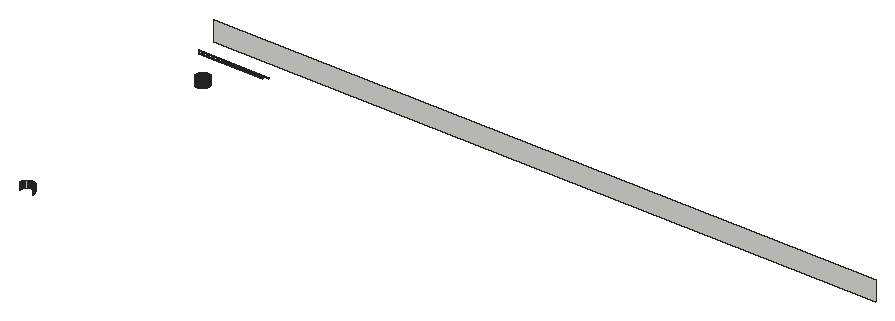
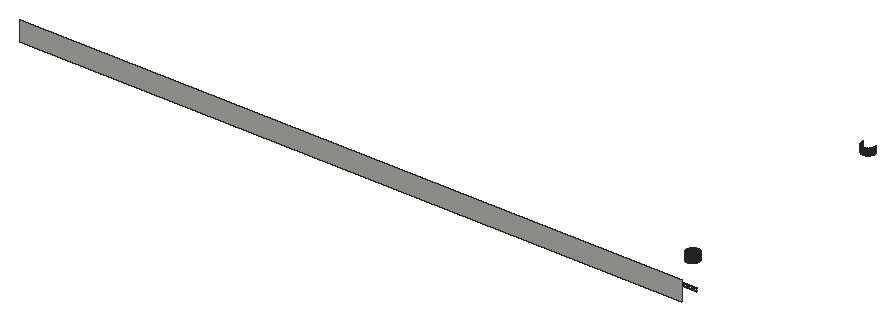
# SketchUp Ruby script. Lengths in inches.
U = 1.inch
M = Sketchup.active_model
def pt(a) = Geom::Point3d.new(a.map { |v| v * U })
def face(e, loops, mat)
  f = e.add_face(loops[0].map { |a| pt(a) })
  loops[1..].each { |l| e.add_face(l.map { |a| pt(a) }).erase! }
  f.material = f.back_material = mat if mat
  f
end
# faces: each face lists its corners as indices into pts; further lists are holes
def faces(e, pts, list, mat = nil) = list.each { |f| face(e, (f[0].is_a?(Array) ? f : [f]).map { |l| l.map { |i| pts[i] } }, mat) }
# xy, xz, yz: faces in a plane at the given z, y or x. An outline is a flat list of corners, or four numbers for a rectangle; further outlines are holes
def ring(l) = l.size == 4 ? [[l[0], l[1]], [l[2], l[1]], [l[2], l[3]], [l[0], l[3]]] : l.each_slice(2).to_a
def flat(e, list, mat, &to3) = list.each { |f| face(e, (f[0].is_a?(Array) ? f : [f]).map { |l| ring(l).map { |u, v| to3.(u, v) } }, mat) }
def xy(e, z, list, mat = nil) = flat(e, list, mat) { |x, y| [x, y, z] }
def xz(e, y, list, mat = nil) = flat(e, list, mat) { |x, z| [x, y, z] }
def yz(e, x, list, mat = nil) = flat(e, list, mat) { |y, z| [x, y, z] }
def lines(e, pts, list) = list.each { |a, b| e.add_line(pt(pts[a]), pt(pts[b])) }
# prism: a flat outline (further loops are holes) pulled along v
def prism(e, loops, v, mat = nil)
  f = face(e, loops, mat); d = Geom::Vector3d.new(v.map { |x| x * U })
  f.pushpull(f.normal.samedirection?(d) ? d.length : -d.length)
end
def box(e, o, s, mat = nil) = prism(e, [[o, [o[0] + s[0], o[1], o[2]], [o[0] + s[0], o[1] + s[1], o[2]], [o[0], o[1] + s[1], o[2]]]], [0, 0, s[2]], mat)
def at(x, y, z, deg = 0) = Geom::Transformation.translation(pt([x, y, z])) * Geom::Transformation.rotation(ORIGIN, Z_AXIS, deg.degrees)
def axes(o, x, y, z) = Geom::Transformation.new([*x, 0, *y, 0, *z, 0, *pt(o).to_a, 1])
def part(name) = M.definitions.add(name)
# library, detail: a bought-in or finely detailed component or shape, given as its bounding box
def library(name, o, s) = part(name).tap { |d| box(d.entities, o, s) }
def detail(e, o, s) = box(e.add_group.entities, o, s)
def put(e, d, t, mat = nil) = e.add_instance(d, t).tap { |i| i.material = mat if mat }
def group(e, t, mat = nil) = e.add_group.tap { |g| g.transformation = t; g.material = mat if mat }.entities
root = M.entities
xz(root,437.5,[[30.34,129,30.42,132],[30.42,129,30.5,132],[30.5,129,30.58,132],[30.58,129,30.66,132]])
xz(root,534,[[30.34,129,30.42,132],[30.42,129,30.5,132],[30.5,129,30.58,132],[30.58,129,30.66,132]])
xz(root,540,[[30.34,129,30.42,132],[30.42,129,30.5,132],[30.5,129,30.58,132],[30.58,129,30.66,132]])
xz(root,553.5,[[15.5,129,45.5,129.5]])
xz(root,555,[[14,129,47,129.5]])
xz(root,564,[[14,129,323,138]])
yz(root,27.5,[[434.34,129,434.42,132],[434.42,129,434.5,132],[434.5,129,434.58,132],[434.58,129,434.66,132],[536.84,129,536.92,132],
  [536.92,129,537,132],[537,129,537.08,132],[537.08,129,537.16,132]])
yz(root,33.5,[[434.34,129,434.42,132],[434.42,129,434.5,132],[434.5,129,434.58,132],[434.58,129,434.66,132],[536.84,129,536.92,132],
  [536.92,129,537,132],[537,129,537.08,132],[537.08,129,537.16,132]])
p = [[27.57,433.875,129],[27.55,433.95,129],[27.55,433.95,132],[27.57,433.875,132],[33.45,433.95,129],[33.43,433.875,129],
  [33.43,433.875,132],[33.45,433.95,132],[27.54,434.03,129],[27.54,434.03,132],[27.53,434.11,129],[27.53,434.11,132],
  [33.46,434.03,129],[33.46,434.03,132],[33.47,434.11,129],[33.47,434.11,132],[27.52,434.1875,129],[27.52,434.1875,132],
  [33.48,434.1875,129],[33.48,434.1875,132],[27.51,434.26,129],[27.51,434.26,132],[33.49,434.26,129],[33.49,434.26,132],
  [27.5,434.34,129],[27.5,434.34,132],[33.5,434.34,129],[33.5,434.34,132],[27.5,434.66,129],[27.51,434.74,129],
  [27.51,434.74,132],[27.5,434.66,132],[27.52,434.8125,129],[27.52,434.8125,132],[33.49,434.74,129],[33.5,434.66,129],
  [33.5,434.66,132],[33.49,434.74,132],[33.48,434.8125,129],[33.48,434.8125,132],[27.53,434.89,129],[27.53,434.89,132],
  [33.47,434.89,129],[33.47,434.89,132],[27.54,434.97,129],[27.54,434.97,132],[33.46,434.97,129],[33.46,434.97,132],
  [27.55,435.05,129],[27.55,435.05,132],[27.57,435.125,129],[27.57,435.125,132],[33.45,435.05,129],[33.45,435.05,132],
  [33.43,435.125,129],[33.43,435.125,132],[27.58,435.2,129],[27.58,435.2,132],[33.42,435.2,129],[33.42,435.2,132],
  [27.6,435.28,129],[27.6,435.28,132],[33.4,435.28,129],[33.4,435.28,132],[27.625,435.35,129],[27.625,435.35,132],
  [33.375,435.35,129],[33.375,435.35,132],[27.65,435.43,129],[27.65,435.43,132],[27.67,435.5,129],[27.67,435.5,132],
  [33.33,435.5,129],[33.35,435.43,129],[33.35,435.43,132],[33.33,435.5,132],[27.7,435.58,129],[27.7,435.58,132],
  [33.3,435.58,129],[33.3,435.58,132],[27.73,435.65,129],[27.73,435.65,132],[27.76,435.72,129],[27.76,435.72,132],
  [33.24,435.72,129],[33.27,435.65,129],[33.27,435.65,132],[33.24,435.72,132],[27.79,435.79,129],[27.79,435.79,132],
  [33.21,435.79,129],[33.21,435.79,132],[27.83,435.86,129],[27.83,435.86,132],[33.17,435.86,129],[33.17,435.86,132],
  [27.86,435.93,129],[27.86,435.93,132],[27.9,436,129],[27.9,436,132],[33.14,435.93,129],[33.14,435.93,132],
  [33.1,436,129],[33.1,436,132],[27.94,436.07,129],[27.94,436.07,132],[33.06,436.07,129],[33.06,436.07,132],
  [27.98,436.13,129],[27.98,436.13,132],[28.03,436.2,129],[28.03,436.2,132],[33.02,436.13,129],[33.02,436.13,132],
  [32.97,436.2,129],[32.97,436.2,132],[28.07,436.26,129],[28.07,436.26,132],[32.93,436.26,129],[32.93,436.26,132],
  [28.12,436.33,129],[28.12,436.33,132],[28.17,436.39,129],[28.17,436.39,132],[32.83,436.39,129],[32.88,436.33,129],
  [32.88,436.33,132],[32.83,436.39,132],[28.22,436.45,129],[28.22,436.45,132],[28.27,436.51,129],[28.27,436.51,132],
  [32.73,436.51,129],[32.78,436.45,129],[32.78,436.45,132],[32.73,436.51,132],[28.32,436.57,129],[28.32,436.57,132],
  [32.68,436.57,129],[32.68,436.57,132],[28.38,436.62,129],[28.38,436.62,132],[28.43,436.68,129],[28.43,436.68,132],
  [32.62,436.62,129],[32.62,436.62,132],[32.57,436.68,129],[32.57,436.68,132],[28.49,436.73,129],[28.49,436.73,132],
  [28.55,436.78,129],[28.55,436.78,132],[32.45,436.78,129],[32.51,436.73,129],[32.51,436.73,132],[32.45,436.78,132],
  [28.61,436.83,129],[28.61,436.83,132],[28.67,436.88,129],[28.67,436.88,132],[32.33,436.88,129],[32.39,436.83,129],
  [32.39,436.83,132],[32.33,436.88,132],[28.74,436.93,129],[28.74,436.93,132],[28.8,436.97,129],[28.8,436.97,132],
  [32.2,436.97,129],[32.26,436.93,129],[32.26,436.93,132],[32.2,436.97,132],[28.87,437.02,129],[28.87,437.02,132],
  [28.93,437.06,129],[28.93,437.06,132],[32.13,437.02,129],[32.13,437.02,132],[32.07,437.06,129],[32.07,437.06,132],
  [29,437.1,129],[29,437.1,132],[29.07,437.14,129],[29.07,437.14,132],[29.14,437.17,129],[29.14,437.17,132],
  [31.93,437.14,129],[32,437.1,129],[32,437.1,132],[31.93,437.14,132],[31.86,437.17,129],[31.86,437.17,132],
  [29.21,437.21,129],[29.21,437.21,132],[29.28,437.24,129],[29.28,437.24,132],[29.35,437.27,129],[29.35,437.27,132],
  [31.65,437.27,129],[31.72,437.24,129],[31.72,437.24,132],[31.65,437.27,132],[31.79,437.21,129],[31.79,437.21,132],
  [29.42,437.3,129],[29.42,437.3,132],[29.5,437.33,129],[29.5,437.33,132],[29.57,437.35,129],[29.57,437.35,132],
  [31.43,437.35,129],[31.5,437.33,129],[31.5,437.33,132],[31.43,437.35,132],[31.58,437.3,129],[31.58,437.3,132],
  [29.65,437.375,129],[29.65,437.375,132],[29.72,437.4,129],[29.72,437.4,132],[29.8,437.42,129],[29.8,437.42,132],
  [29.875,437.43,129],[29.875,437.43,132],[29.95,437.45,129],[29.95,437.45,132],[30.03,437.46,129],[30.03,437.46,132],
  [31.05,437.45,129],[31.125,437.43,129],[31.125,437.43,132],[31.05,437.45,132],[30.97,437.46,129],[30.97,437.46,132],
  [31.2,437.42,129],[31.2,437.42,132],[31.28,437.4,129],[31.28,437.4,132],[31.35,437.375,129],[31.35,437.375,132],
  [30.11,437.47,129],[30.11,437.47,132],[30.1875,437.48,129],[30.1875,437.48,132],[30.26,437.49,129],[30.26,437.49,132],
  [30.34,437.5,129],[30.34,437.5,132],[30.74,437.49,129],[30.8125,437.48,129],[30.8125,437.48,132],[30.74,437.49,132],
  [30.66,437.5,129],[30.66,437.5,132],[30.89,437.47,129],[30.89,437.47,132],[30.11,534.03,129],[30.03,534.04,129],
  [30.03,534.04,132],[30.11,534.03,132],[29.95,534.05,129],[29.95,534.05,132],[30.1875,534.02,129],[30.1875,534.02,132],
  [30.26,534.01,129],[30.26,534.01,132],[30.34,534,129],[30.34,534,132],[30.74,534.01,129],[30.66,534,129],
  [30.66,534,132],[30.74,534.01,132],[30.8125,534.02,129],[30.8125,534.02,132],[30.89,534.03,129],[30.89,534.03,132],
  [30.97,534.04,129],[30.97,534.04,132],[31.05,534.05,129],[31.05,534.05,132],[29.57,534.15,129],[29.5,534.17,129],
  [29.5,534.17,132],[29.57,534.15,132],[29.72,534.1,129],[29.65,534.125,129],[29.65,534.125,132],[29.72,534.1,132],
  [29.8,534.08,129],[29.8,534.08,132],[29.875,534.07,129],[29.875,534.07,132],[31.125,534.07,129],[31.125,534.07,132],
  [31.2,534.08,129],[31.2,534.08,132],[31.28,534.1,129],[31.28,534.1,132],[31.35,534.125,129],[31.35,534.125,132],
  [31.43,534.15,129],[31.43,534.15,132],[31.5,534.17,129],[31.5,534.17,132],[29.35,534.23,129],[29.28,534.26,129],
  [29.28,534.26,132],[29.35,534.23,132],[29.42,534.2,129],[29.42,534.2,132],[31.58,534.2,129],[31.58,534.2,132],
  [31.65,534.23,129],[31.65,534.23,132],[31.72,534.26,129],[31.72,534.26,132],[29.21,534.29,129],[29.14,534.33,129],
  [29.14,534.33,132],[29.21,534.29,132],[29.07,534.36,129],[29.07,534.36,132],[31.79,534.29,129],[31.79,534.29,132],
  [31.86,534.33,129],[31.86,534.33,132],[31.93,534.36,129],[31.93,534.36,132],[29,534.4,129],[28.93,534.44,129],
  [28.93,534.44,132],[29,534.4,132],[28.87,534.48,129],[28.87,534.48,132],[32,534.4,129],[32,534.4,132],
  [32.07,534.44,129],[32.07,534.44,132],[32.13,534.48,129],[32.13,534.48,132],[28.8,534.53,129],[28.74,534.57,129],
  [28.74,534.57,132],[28.8,534.53,132],[32.2,534.53,129],[32.2,534.53,132],[32.26,534.57,129],[32.26,534.57,132],
  [28.67,534.62,129],[28.61,534.67,129],[28.61,534.67,132],[28.67,534.62,132],[32.33,534.62,129],[32.33,534.62,132],
  [32.39,534.67,129],[32.39,534.67,132],[28.55,534.72,129],[28.49,534.77,129],[28.49,534.77,132],[28.55,534.72,132],
  [32.45,534.72,129],[32.45,534.72,132],[32.51,534.77,129],[32.51,534.77,132],[28.43,534.82,129],[28.43,534.82,132],
  [28.38,534.88,129],[28.38,534.88,132],[32.57,534.82,129],[32.57,534.82,132],[32.62,534.88,129],[32.62,534.88,132],
  [28.32,534.93,129],[28.32,534.93,132],[28.27,534.99,129],[28.27,534.99,132],[32.68,534.93,129],[32.68,534.93,132],
  [32.73,534.99,129],[32.73,534.99,132],[28.22,535.05,129],[28.22,535.05,132],[32.78,535.05,129],[32.78,535.05,132],
  [28.17,535.11,129],[28.12,535.17,129],[28.12,535.17,132],[28.17,535.11,132],[32.83,535.11,129],[32.83,535.11,132],
  [32.88,535.17,129],[32.88,535.17,132],[28.07,535.24,129],[28.03,535.3,129],[28.03,535.3,132],[28.07,535.24,132],
  [32.93,535.24,129],[32.93,535.24,132],[32.97,535.3,129],[32.97,535.3,132],[27.98,535.37,129],[27.98,535.37,132],
  [33.02,535.37,129],[33.02,535.37,132],[27.94,535.43,129],[27.94,535.43,132],[27.9,535.5,129],[27.9,535.5,132],
  [33.06,535.43,129],[33.06,535.43,132],[33.1,535.5,129],[33.1,535.5,132],[27.86,535.57,129],[27.86,535.57,132],
  [33.14,535.57,129],[33.14,535.57,132],[27.83,535.64,129],[27.83,535.64,132],[27.79,535.71,129],[27.79,535.71,132],
  [33.17,535.64,129],[33.17,535.64,132],[33.21,535.71,129],[33.21,535.71,132],[27.76,535.78,129],[27.76,535.78,132],
  [33.24,535.78,129],[33.24,535.78,132],[27.73,535.85,129],[27.73,535.85,132],[33.27,535.85,129],[33.27,535.85,132],
  [27.7,535.92,129],[27.7,535.92,132],[27.67,536,129],[27.67,536,132],[33.3,535.92,129],[33.3,535.92,132],
  [33.33,536,129],[33.33,536,132],[27.65,536.07,129],[27.65,536.07,132],[33.35,536.07,129],[33.35,536.07,132],
  [27.625,536.15,129],[27.625,536.15,132],[27.6,536.22,129],[27.6,536.22,132],[33.375,536.15,129],[33.375,536.15,132],
  [33.4,536.22,129],[33.4,536.22,132],[27.58,536.3,129],[27.58,536.3,132],[33.42,536.3,129],[33.42,536.3,132],
  [27.57,536.375,129],[27.57,536.375,132],[33.43,536.375,129],[33.43,536.375,132],[27.55,536.45,129],[27.55,536.45,132],
  [33.45,536.45,129],[33.45,536.45,132],[27.54,536.53,129],[27.54,536.53,132],[27.53,536.61,129],[27.53,536.61,132],
  [33.46,536.53,129],[33.46,536.53,132],[33.47,536.61,129],[33.47,536.61,132],[27.52,536.6875,129],[27.52,536.6875,132],
  [33.48,536.6875,129],[33.48,536.6875,132],[27.51,536.76,129],[27.51,536.76,132],[33.49,536.76,129],[33.49,536.76,132],
  [27.5,536.84,129],[27.5,536.84,132],[33.5,536.84,129],[33.5,536.84,132],[27.5,537.16,129],[27.51,537.24,129],
  [27.51,537.24,132],[27.5,537.16,132],[27.52,537.3125,129],[27.52,537.3125,132],[33.49,537.24,129],[33.5,537.16,129],
  [33.5,537.16,132],[33.49,537.24,132],[33.48,537.3125,129],[33.48,537.3125,132],[27.53,537.39,129],[27.53,537.39,132],
  [33.47,537.39,129],[33.47,537.39,132],[27.54,537.47,129],[27.54,537.47,132],[33.46,537.47,129],[33.46,537.47,132],
  [27.55,537.55,129],[27.55,537.55,132],[27.57,537.625,129],[27.57,537.625,132],[33.45,537.55,129],[33.45,537.55,132],
  [33.43,537.625,129],[33.43,537.625,132],[27.58,537.7,129],[27.58,537.7,132],[33.42,537.7,129],[33.42,537.7,132],
  [27.6,537.78,129],[27.6,537.78,132],[33.4,537.78,129],[33.4,537.78,132],[27.625,537.85,129],[27.625,537.85,132],
  [33.375,537.85,129],[33.375,537.85,132],[27.65,537.93,129],[27.65,537.93,132],[27.67,538,129],[27.67,538,132],
  [33.33,538,129],[33.35,537.93,129],[33.35,537.93,132],[33.33,538,132],[27.7,538.08,129],[27.7,538.08,132],
  [33.3,538.08,129],[33.3,538.08,132],[27.73,538.15,129],[27.73,538.15,132],[27.76,538.22,129],[27.76,538.22,132],
  [33.24,538.22,129],[33.27,538.15,129],[33.27,538.15,132],[33.24,538.22,132],[27.79,538.29,129],[27.79,538.29,132],
  [33.21,538.29,129],[33.21,538.29,132],[27.83,538.36,129],[27.83,538.36,132],[33.17,538.36,129],[33.17,538.36,132],
  [27.86,538.43,129],[27.86,538.43,132],[27.9,538.5,129],[27.9,538.5,132],[33.14,538.43,129],[33.14,538.43,132],
  [33.1,538.5,129],[33.1,538.5,132],[27.94,538.57,129],[27.94,538.57,132],[33.06,538.57,129],[33.06,538.57,132],
  [27.98,538.63,129],[27.98,538.63,132],[28.03,538.7,129],[28.03,538.7,132],[33.02,538.63,129],[33.02,538.63,132],
  [32.97,538.7,129],[32.97,538.7,132],[28.07,538.76,129],[28.07,538.76,132],[32.93,538.76,129],[32.93,538.76,132],
  [28.12,538.83,129],[28.12,538.83,132],[28.17,538.89,129],[28.17,538.89,132],[32.83,538.89,129],[32.88,538.83,129],
  [32.88,538.83,132],[32.83,538.89,132],[28.22,538.95,129],[28.22,538.95,132],[28.27,539.01,129],[28.27,539.01,132],
  [32.73,539.01,129],[32.78,538.95,129],[32.78,538.95,132],[32.73,539.01,132],[28.32,539.07,129],[28.32,539.07,132],
  [32.68,539.07,129],[32.68,539.07,132],[28.38,539.12,129],[28.38,539.12,132],[28.43,539.18,129],[28.43,539.18,132],
  [32.62,539.12,129],[32.62,539.12,132],[32.57,539.18,129],[32.57,539.18,132],[28.49,539.23,129],[28.49,539.23,132],
  [28.55,539.28,129],[28.55,539.28,132],[32.45,539.28,129],[32.51,539.23,129],[32.51,539.23,132],[32.45,539.28,132],
  [28.61,539.33,129],[28.61,539.33,132],[28.67,539.38,129],[28.67,539.38,132],[32.33,539.38,129],[32.39,539.33,129],
  [32.39,539.33,132],[32.33,539.38,132],[28.74,539.43,129],[28.74,539.43,132],[28.8,539.47,129],[28.8,539.47,132],
  [32.2,539.47,129],[32.26,539.43,129],[32.26,539.43,132],[32.2,539.47,132],[28.87,539.52,129],[28.87,539.52,132],
  [28.93,539.56,129],[28.93,539.56,132],[32.13,539.52,129],[32.13,539.52,132],[32.07,539.56,129],[32.07,539.56,132],
  [29,539.6,129],[29,539.6,132],[29.07,539.64,129],[29.07,539.64,132],[29.14,539.67,129],[29.14,539.67,132],
  [31.93,539.64,129],[32,539.6,129],[32,539.6,132],[31.93,539.64,132],[31.86,539.67,129],[31.86,539.67,132],
  [29.21,539.71,129],[29.21,539.71,132],[29.28,539.74,129],[29.28,539.74,132],[29.35,539.77,129],[29.35,539.77,132],
  [31.65,539.77,129],[31.72,539.74,129],[31.72,539.74,132],[31.65,539.77,132],[31.79,539.71,129],[31.79,539.71,132],
  [29.42,539.8,129],[29.42,539.8,132],[29.5,539.83,129],[29.5,539.83,132],[29.57,539.85,129],[29.57,539.85,132],
  [31.43,539.85,129],[31.5,539.83,129],[31.5,539.83,132],[31.43,539.85,132],[31.58,539.8,129],[31.58,539.8,132],
  [29.65,539.875,129],[29.65,539.875,132],[29.72,539.9,129],[29.72,539.9,132],[29.8,539.92,129],[29.8,539.92,132],
  [29.875,539.93,129],[29.875,539.93,132],[29.95,539.95,129],[29.95,539.95,132],[30.03,539.96,129],[30.03,539.96,132],
  [31.05,539.95,129],[31.125,539.93,129],[31.125,539.93,132],[31.05,539.95,132],[30.97,539.96,129],[30.97,539.96,132],
  [31.2,539.92,129],[31.2,539.92,132],[31.28,539.9,129],[31.28,539.9,132],[31.35,539.875,129],[31.35,539.875,132],
  [30.11,539.97,129],[30.11,539.97,132],[30.1875,539.98,129],[30.1875,539.98,132],[30.26,539.99,129],[30.26,539.99,132],
  [30.34,540,129],[30.34,540,132],[30.74,539.99,129],[30.8125,539.98,129],[30.8125,539.98,132],[30.74,539.99,132],
  [30.66,540,129],[30.66,540,132],[30.89,539.97,129],[30.89,539.97,132]]
faces(root,p,[[0,1,2,3],[4,5,6,7],[1,8,9,2],[8,10,11,9],[12,4,7,13],[14,12,13,15],[10,16,17,11],[18,14,15,19],
  [16,20,21,17],[22,18,19,23],[20,24,25,21],[26,22,23,27],[28,29,30,31],[29,32,33,30],[34,35,36,37],[38,34,37,39],
  [32,40,41,33],[42,38,39,43],[40,44,45,41],[46,42,43,47],[44,48,49,45],[48,50,51,49],[52,46,47,53],[54,52,53,55],
  [50,56,57,51],[58,54,55,59],[56,60,61,57],[62,58,59,63],[60,64,65,61],[66,62,63,67],[64,68,69,65],[68,70,71,69],
  [72,73,74,75],[73,66,67,74],[70,76,77,71],[78,72,75,79],[76,80,81,77],[80,82,83,81],[84,85,86,87],[85,78,79,86],
  [82,88,89,83],[90,84,87,91],[88,92,93,89],[94,90,91,95],[92,96,97,93],[96,98,99,97],[100,94,95,101],[102,100,101,103],
  [98,104,105,99],[106,102,103,107],[104,108,109,105],[108,110,111,109],[112,106,107,113],[114,112,113,115],[110,116,117,111],[118,114,115,119],
  [116,120,121,117],[120,122,123,121],[124,125,126,127],[125,118,119,126],[122,128,129,123],[128,130,131,129],[132,133,134,135],[133,124,127,134],
  [130,136,137,131],[138,132,135,139],[136,140,141,137],[140,142,143,141],[144,138,139,145],[146,144,145,147],[142,148,149,143],[148,150,151,149],
  [152,153,154,155],[153,146,147,154],[150,156,157,151],[156,158,159,157],[160,161,162,163],[161,152,155,162],[158,164,165,159],[164,166,167,165],
  [168,169,170,171],[169,160,163,170],[166,172,173,167],[172,174,175,173],[176,168,171,177],[178,176,177,179],[174,180,181,175],[180,182,183,181],
  [182,184,185,183],[186,187,188,189],[190,186,189,191],[187,178,179,188],[184,192,193,185],[192,194,195,193],[194,196,197,195],[198,199,200,201],
  [199,202,203,200],[202,190,191,203],[196,204,205,197],[204,206,207,205],[206,208,209,207],[210,211,212,213],[211,214,215,212],[214,198,201,215],
  [208,216,217,209],[216,218,219,217],[218,220,221,219],[220,222,223,221],[222,224,225,223],[224,226,227,225],[228,229,230,231],[232,228,231,233],
  [229,234,235,230],[234,236,237,235],[236,238,239,237],[238,210,213,239],[226,240,241,227],[240,242,243,241],[242,244,245,243],[244,246,247,245],
  [248,249,250,251],[252,248,251,253],[249,254,255,250],[254,232,233,255],[256,257,258,259],[257,260,261,258],[262,256,259,263],[264,262,263,265],
  [266,264,265,267],[268,269,270,271],[272,268,271,273],[274,272,273,275],[276,274,275,277],[278,276,277,279],[280,281,282,283],[284,285,286,287],
  [285,280,283,286],[288,284,287,289],[290,288,289,291],[260,290,291,261],[292,278,279,293],[294,292,293,295],[296,294,295,297],[298,296,297,299],
  [300,298,299,301],[302,300,301,303],[304,305,306,307],[281,308,309,282],[308,304,307,309],[310,302,303,311],[312,310,311,313],[314,312,313,315],
  [316,317,318,319],[317,320,321,318],[305,316,319,306],[322,314,315,323],[324,322,323,325],[326,324,325,327],[328,329,330,331],[329,332,333,330],
  [320,328,331,321],[334,326,327,335],[336,334,335,337],[338,336,337,339],[340,341,342,343],[332,340,343,333],[344,338,339,345],[346,344,345,347],
  [348,349,350,351],[341,348,351,342],[352,346,347,353],[354,352,353,355],[356,357,358,359],[349,356,359,350],[360,354,355,361],[362,360,361,363],
  [357,364,365,358],[364,366,367,365],[368,362,363,369],[370,368,369,371],[366,372,373,367],[372,374,375,373],[376,370,371,377],[378,376,377,379],
  [374,380,381,375],[382,378,379,383],[384,385,386,387],[380,384,387,381],[388,382,383,389],[390,388,389,391],[392,393,394,395],[385,392,395,386],
  [396,390,391,397],[398,396,397,399],[393,400,401,394],[402,398,399,403],[400,404,405,401],[404,406,407,405],[408,402,403,409],[410,408,409,411],
  [406,412,413,407],[414,410,411,415],[412,416,417,413],[416,418,419,417],[420,414,415,421],[422,420,421,423],[418,424,425,419],[426,422,423,427],
  [424,428,429,425],[430,426,427,431],[428,432,433,429],[432,434,435,433],[436,430,431,437],[438,436,437,439],[434,440,441,435],[442,438,439,443],
  [440,444,445,441],[444,446,447,445],[448,442,443,449],[450,448,449,451],[446,452,453,447],[454,450,451,455],[452,456,457,453],[458,454,455,459],
  [456,460,461,457],[462,458,459,463],[460,464,465,461],[464,466,467,465],[468,462,463,469],[470,468,469,471],[466,472,473,467],[474,470,471,475],
  [472,476,477,473],[478,474,475,479],[476,480,481,477],[482,478,479,483],[484,485,486,487],[485,488,489,486],[490,491,492,493],[494,490,493,495],
  [488,496,497,489],[498,494,495,499],[496,500,501,497],[502,498,499,503],[500,504,505,501],[504,506,507,505],[508,502,503,509],[510,508,509,511],
  [506,512,513,507],[514,510,511,515],[512,516,517,513],[518,514,515,519],[516,520,521,517],[522,518,519,523],[520,524,525,521],[524,526,527,525],
  [528,529,530,531],[529,522,523,530],[526,532,533,527],[534,528,531,535],[532,536,537,533],[536,538,539,537],[540,541,542,543],[541,534,535,542],
  [538,544,545,539],[546,540,543,547],[544,548,549,545],[550,546,547,551],[548,552,553,549],[552,554,555,553],[556,550,551,557],[558,556,557,559],
  [554,560,561,555],[562,558,559,563],[560,564,565,561],[564,566,567,565],[568,562,563,569],[570,568,569,571],[566,572,573,567],[574,570,571,575],
  [572,576,577,573],[576,578,579,577],[580,581,582,583],[581,574,575,582],[578,584,585,579],[584,586,587,585],[588,589,590,591],[589,580,583,590],
  [586,592,593,587],[594,588,591,595],[592,596,597,593],[596,598,599,597],[600,594,595,601],[602,600,601,603],[598,604,605,599],[604,606,607,605],
  [608,609,610,611],[609,602,603,610],[606,612,613,607],[612,614,615,613],[616,617,618,619],[617,608,611,618],[614,620,621,615],[620,622,623,621],
  [624,625,626,627],[625,616,619,626],[622,628,629,623],[628,630,631,629],[632,624,627,633],[634,632,633,635],[630,636,637,631],[636,638,639,637],
  [638,640,641,639],[642,643,644,645],[646,642,645,647],[643,634,635,644],[640,648,649,641],[648,650,651,649],[650,652,653,651],[654,655,656,657],
  [655,658,659,656],[658,646,647,659],[652,660,661,653],[660,662,663,661],[662,664,665,663],[666,667,668,669],[667,670,671,668],[670,654,657,671],
  [664,672,673,665],[672,674,675,673],[674,676,677,675],[676,678,679,677],[678,680,681,679],[680,682,683,681],[684,685,686,687],[688,684,687,689],
  [685,690,691,686],[690,692,693,691],[692,694,695,693],[694,666,669,695],[682,696,697,683],[696,698,699,697],[698,700,701,699],[700,702,703,701],
  [704,705,706,707],[708,704,707,709],[705,710,711,706],[710,688,689,711]])
